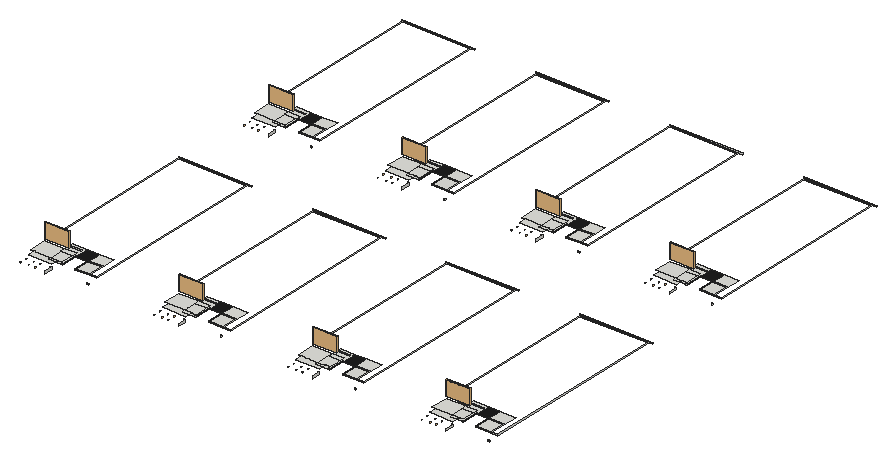
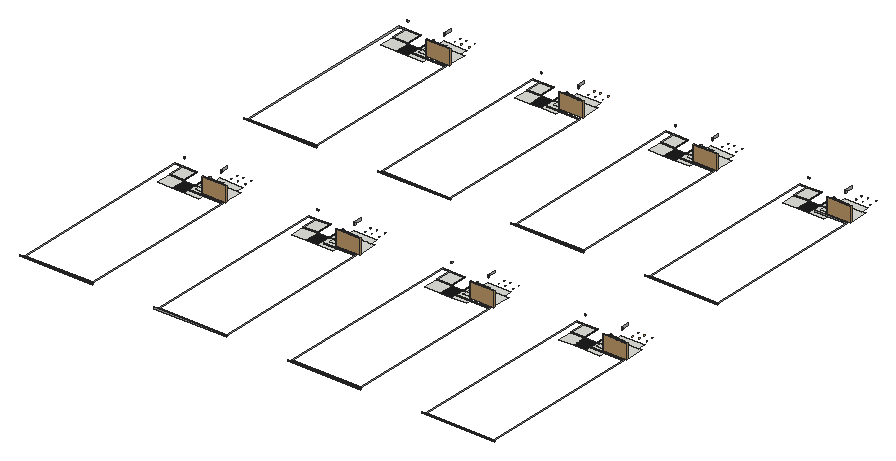
# SketchUp Ruby script. Lengths in inches.
U = 1.inch
M = Sketchup.active_model
def pt(a) = Geom::Point3d.new(a.map { |v| v * U })
def face(e, loops, mat)
  f = e.add_face(loops[0].map { |a| pt(a) })
  loops[1..].each { |l| e.add_face(l.map { |a| pt(a) }).erase! }
  f.material = f.back_material = mat if mat
  f
end
# faces: each face lists its corners as indices into pts; further lists are holes
def faces(e, pts, list, mat = nil) = list.each { |f| face(e, (f[0].is_a?(Array) ? f : [f]).map { |l| l.map { |i| pts[i] } }, mat) }
# xy, xz, yz: faces in a plane at the given z, y or x. An outline is a flat list of corners, or four numbers for a rectangle; further outlines are holes
def ring(l) = l.size == 4 ? [[l[0], l[1]], [l[2], l[1]], [l[2], l[3]], [l[0], l[3]]] : l.each_slice(2).to_a
def flat(e, list, mat, &to3) = list.each { |f| face(e, (f[0].is_a?(Array) ? f : [f]).map { |l| ring(l).map { |u, v| to3.(u, v) } }, mat) }
def xy(e, z, list, mat = nil) = flat(e, list, mat) { |x, y| [x, y, z] }
def xz(e, y, list, mat = nil) = flat(e, list, mat) { |x, z| [x, y, z] }
def yz(e, x, list, mat = nil) = flat(e, list, mat) { |y, z| [x, y, z] }
def lines(e, pts, list) = list.each { |a, b| e.add_line(pt(pts[a]), pt(pts[b])) }
# prism: a flat outline (further loops are holes) pulled along v
def prism(e, loops, v, mat = nil)
  f = face(e, loops, mat); d = Geom::Vector3d.new(v.map { |x| x * U })
  f.pushpull(f.normal.samedirection?(d) ? d.length : -d.length)
end
def box(e, o, s, mat = nil) = prism(e, [[o, [o[0] + s[0], o[1], o[2]], [o[0] + s[0], o[1] + s[1], o[2]], [o[0], o[1] + s[1], o[2]]]], [0, 0, s[2]], mat)
def at(x, y, z, deg = 0) = Geom::Transformation.translation(pt([x, y, z])) * Geom::Transformation.rotation(ORIGIN, Z_AXIS, deg.degrees)
def axes(o, x, y, z) = Geom::Transformation.new([*x, 0, *y, 0, *z, 0, *pt(o).to_a, 1])
def part(name) = M.definitions.add(name)
# library, detail: a bought-in or finely detailed component or shape, given as its bounding box
def library(name, o, s) = part(name).tap { |d| box(d.entities, o, s) }
def detail(e, o, s) = box(e.add_group.entities, o, s)
def put(e, d, t, mat = nil) = e.add_instance(d, t).tap { |i| i.material = mat if mat }
def group(e, t, mat = nil) = e.add_group.tap { |g| g.transformation = t; g.material = mat if mat }.entities
root = M.entities
M.materials.add("[Color M08]").color = [30, 30, 30]
M.materials.add("[Field Square Tile]").color = [211, 167, 108]
c1 = library("Curtains",[0,0,0],[121.73,8.19,117.22])
xy(root,252.4375,[[357.2,526.75,356.76,526.8125,356.35,526.98,356,527.25,355.74,527.6,355.57,528,355.51,528.44,355.57,528.88,355.74,529.28,356,529.63,356.35,529.9,356.76,530.07,357.2,530.13,357.63,530.07,358.04,529.9,358.39,529.63,358.66,529.28,358.83,528.88,358.88,528.44,358.83,528,358.66,527.6,358.39,527.25,358.04,526.98,357.63,526.8125],[1235.95,526.75,1235.51,526.8125,1235.1,526.98,1234.75,527.25,1234.49,527.6,1234.32,528,1234.26,528.44,1234.32,528.88,1234.49,529.28,1234.75,529.63,1235.1,529.9,1235.51,530.07,1235.95,530.13,1236.38,530.07,1236.79,529.9,1237.14,529.63,1237.41,529.28,1237.58,528.88,1237.63,528.44,1237.58,528,1237.41,527.6,1237.14,527.25,1236.79,526.98,1236.38,526.8125],[2114.7,526.75,2114.26,526.8125,2113.85,526.98,2113.5,527.25,2113.24,527.6,2113.07,528,2113.01,528.44,2113.07,528.88,2113.24,529.28,2113.5,529.63,2113.85,529.9,2114.26,530.07,2114.7,530.13,2115.13,530.07,2115.54,529.9,2115.89,529.63,2116.16,529.28,2116.33,528.88,2116.38,528.44,2116.33,528,2116.16,527.6,2115.89,527.25,2115.54,526.98,2115.13,526.8125],[2993.45,526.75,2993.01,526.8125,2992.6,526.98,2992.25,527.25,2991.99,527.6,2991.82,528,2991.76,528.44,2991.82,528.88,2991.99,529.28,2992.25,529.63,2992.6,529.9,2993.01,530.07,2993.45,530.13,2993.88,530.07,2994.29,529.9,2994.64,529.63,2994.91,529.28,2995.08,528.88,2995.13,528.44,2995.08,528,2994.91,527.6,2994.64,527.25,2994.29,526.98,2993.88,526.8125],[357.2,2362.38,356.76,2362.4375,356.35,2362.6,356,2362.87,355.74,2363.22,355.57,2363.63,355.51,2364.07,355.57,2364.5,355.74,2364.91,356,2365.26,356.35,2365.53,356.76,2365.7,357.2,2365.75,357.63,2365.7,358.04,2365.53,358.39,2365.26,358.66,2364.91,358.83,2364.5,358.88,2364.07,358.83,2363.63,358.66,2363.22,358.39,2362.87,358.04,2362.6,357.63,2362.4375],
  [1235.95,2362.38,1235.51,2362.4375,1235.1,2362.6,1234.75,2362.87,1234.49,2363.22,1234.32,2363.63,1234.26,2364.07,1234.32,2364.5,1234.49,2364.91,1234.75,2365.26,1235.1,2365.53,1235.51,2365.7,1235.95,2365.75,1236.38,2365.7,1236.79,2365.53,1237.14,2365.26,1237.41,2364.91,1237.58,2364.5,1237.63,2364.07,1237.58,2363.63,1237.41,2363.22,1237.14,2362.87,1236.79,2362.6,1236.38,2362.4375],[2114.7,2362.38,2114.26,2362.4375,2113.85,2362.6,2113.5,2362.87,2113.24,2363.22,2113.07,2363.63,2113.01,2364.07,2113.07,2364.5,2113.24,2364.91,2113.5,2365.26,2113.85,2365.53,2114.26,2365.7,2114.7,2365.75,2115.13,2365.7,2115.54,2365.53,2115.89,2365.26,2116.16,2364.91,2116.33,2364.5,2116.38,2364.07,2116.33,2363.63,2116.16,2363.22,2115.89,2362.87,2115.54,2362.6,2115.13,2362.4375],[2993.45,2362.38,2993.01,2362.4375,2992.6,2362.6,2992.25,2362.87,2991.99,2363.22,2991.82,2363.63,2991.76,2364.07,2991.82,2364.5,2991.99,2364.91,2992.25,2365.26,2992.6,2365.53,2993.01,2365.7,2993.45,2365.75,2993.88,2365.7,2994.29,2365.53,2994.64,2365.26,2994.91,2364.91,2995.08,2364.5,2995.13,2364.07,2995.08,2363.63,2994.91,2363.22,2994.64,2362.87,2994.29,2362.6,2993.88,2362.4375]],"[Field Square Tile]")
xy(root,252.5,[[266.8,476.64,266.3125,476.71,265.86,476.89,265.47,477.19,265.17,477.58,264.99,478.03,264.92,478.52,264.99,479,265.17,479.45,265.47,479.84,265.86,480.14,266.3125,480.33,266.8,480.39,267.28,480.33,267.74,480.14,268.125,479.84,268.42,479.45,268.61,479,268.67,478.52,268.61,478.03,268.42,477.58,268.125,477.19,267.74,476.89,267.28,476.71],[1145.55,476.64,1145.0625,476.71,1144.61,476.89,1144.22,477.19,1143.92,477.58,1143.74,478.03,1143.67,478.52,1143.74,479,1143.92,479.45,1144.22,479.84,1144.61,480.14,1145.0625,480.33,1145.55,480.39,1146.03,480.33,1146.49,480.14,1146.875,479.84,1147.17,479.45,1147.36,479,1147.42,478.52,1147.36,478.03,1147.17,477.58,1146.875,477.19,1146.49,476.89,1146.03,476.71],[2024.3,476.64,2023.8125,476.71,2023.36,476.89,2022.97,477.19,2022.67,477.58,2022.49,478.03,2022.42,478.52,2022.49,479,2022.67,479.45,2022.97,479.84,2023.36,480.14,2023.8125,480.33,2024.3,480.39,2024.78,480.33,2025.24,480.14,2025.625,479.84,2025.92,479.45,2026.11,479,2026.17,478.52,2026.11,478.03,2025.92,477.58,2025.625,477.19,2025.24,476.89,2024.78,476.71],[2903.05,476.64,2902.5625,476.71,2902.11,476.89,2901.72,477.19,2901.42,477.58,2901.24,478.03,2901.17,478.52,2901.24,479,2901.42,479.45,2901.72,479.84,2902.11,480.14,2902.5625,480.33,2903.05,480.39,2903.53,480.33,2903.99,480.14,2904.375,479.84,2904.67,479.45,2904.86,479,2904.92,478.52,2904.86,478.03,2904.67,477.58,2904.375,477.19,2903.99,476.89,2903.53,476.71],[317.24,479.77,316.75,479.83,316.3,480.02,315.91,480.32,315.61,480.7,315.42,481.16,315.36,481.64,315.42,482.13,315.61,482.58,315.91,482.97,316.3,483.27,316.75,483.45,317.24,483.52,317.72,483.45,318.17,483.27,318.5625,482.97,318.86,482.58,319.05,482.13,319.11,481.64,319.05,481.16,318.86,480.7,318.5625,480.32,318.17,480.02,317.72,479.83],
  [1195.99,479.77,1195.5,479.83,1195.05,480.02,1194.66,480.32,1194.36,480.7,1194.17,481.16,1194.11,481.64,1194.17,482.13,1194.36,482.58,1194.66,482.97,1195.05,483.27,1195.5,483.45,1195.99,483.52,1196.47,483.45,1196.92,483.27,1197.3125,482.97,1197.61,482.58,1197.8,482.13,1197.86,481.64,1197.8,481.16,1197.61,480.7,1197.3125,480.32,1196.92,480.02,1196.47,479.83],[2074.74,479.77,2074.25,479.83,2073.8,480.02,2073.41,480.32,2073.11,480.7,2072.92,481.16,2072.86,481.64,2072.92,482.13,2073.11,482.58,2073.41,482.97,2073.8,483.27,2074.25,483.45,2074.74,483.52,2075.22,483.45,2075.67,483.27,2076.0625,482.97,2076.36,482.58,2076.55,482.13,2076.61,481.64,2076.55,481.16,2076.36,480.7,2076.0625,480.32,2075.67,480.02,2075.22,479.83],[2953.49,479.77,2953,479.83,2952.55,480.02,2952.16,480.32,2951.86,480.7,2951.67,481.16,2951.61,481.64,2951.67,482.13,2951.86,482.58,2952.16,482.97,2952.55,483.27,2953,483.45,2953.49,483.52,2953.97,483.45,2954.42,483.27,2954.8125,482.97,2955.11,482.58,2955.3,482.13,2955.36,481.64,2955.3,481.16,2955.11,480.7,2954.8125,480.32,2954.42,480.02,2953.97,479.83],[266.8,522.58,266.3125,522.64,265.86,522.83,265.47,523.13,265.17,523.52,264.99,523.97,264.92,524.45,264.99,524.94,265.17,525.39,265.47,525.78,265.86,526.08,266.3125,526.27,266.8,526.33,267.28,526.27,267.74,526.08,268.125,525.78,268.42,525.39,268.61,524.94,268.67,524.45,268.61,523.97,268.42,523.52,268.125,523.13,267.74,522.83,267.28,522.64],[317.24,522.58,316.75,522.64,316.3,522.83,315.91,523.13,315.61,523.52,315.42,523.97,315.36,524.45,315.42,524.94,315.61,525.39,315.91,525.78,316.3,526.08,316.75,526.27,317.24,526.33,317.72,526.27,318.17,526.08,318.5625,525.78,318.86,525.39,319.05,524.94,319.11,524.45,319.05,523.97,318.86,523.52,318.5625,523.13,318.17,522.83,317.72,522.64],
  [1145.55,522.58,1145.0625,522.64,1144.61,522.83,1144.22,523.13,1143.92,523.52,1143.74,523.97,1143.67,524.45,1143.74,524.94,1143.92,525.39,1144.22,525.78,1144.61,526.08,1145.0625,526.27,1145.55,526.33,1146.03,526.27,1146.49,526.08,1146.875,525.78,1147.17,525.39,1147.36,524.94,1147.42,524.45,1147.36,523.97,1147.17,523.52,1146.875,523.13,1146.49,522.83,1146.03,522.64],[1195.99,522.58,1195.5,522.64,1195.05,522.83,1194.66,523.13,1194.36,523.52,1194.17,523.97,1194.11,524.45,1194.17,524.94,1194.36,525.39,1194.66,525.78,1195.05,526.08,1195.5,526.27,1195.99,526.33,1196.47,526.27,1196.92,526.08,1197.3125,525.78,1197.61,525.39,1197.8,524.94,1197.86,524.45,1197.8,523.97,1197.61,523.52,1197.3125,523.13,1196.92,522.83,1196.47,522.64],[2024.3,522.58,2023.8125,522.64,2023.36,522.83,2022.97,523.13,2022.67,523.52,2022.49,523.97,2022.42,524.45,2022.49,524.94,2022.67,525.39,2022.97,525.78,2023.36,526.08,2023.8125,526.27,2024.3,526.33,2024.78,526.27,2025.24,526.08,2025.625,525.78,2025.92,525.39,2026.11,524.94,2026.17,524.45,2026.11,523.97,2025.92,523.52,2025.625,523.13,2025.24,522.83,2024.78,522.64],[2074.74,522.58,2074.25,522.64,2073.8,522.83,2073.41,523.13,2073.11,523.52,2072.92,523.97,2072.86,524.45,2072.92,524.94,2073.11,525.39,2073.41,525.78,2073.8,526.08,2074.25,526.27,2074.74,526.33,2075.22,526.27,2075.67,526.08,2076.0625,525.78,2076.36,525.39,2076.55,524.94,2076.61,524.45,2076.55,523.97,2076.36,523.52,2076.0625,523.13,2075.67,522.83,2075.22,522.64],[2903.05,522.58,2902.5625,522.64,2902.11,522.83,2901.72,523.13,2901.42,523.52,2901.24,523.97,2901.17,524.45,2901.24,524.94,2901.42,525.39,2901.72,525.78,2902.11,526.08,2902.5625,526.27,2903.05,526.33,2903.53,526.27,2903.99,526.08,2904.375,525.78,2904.67,525.39,2904.86,524.94,2904.92,524.45,2904.86,523.97,2904.67,523.52,2904.375,523.13,2903.99,522.83,2903.53,522.64],
  [2953.49,522.58,2953,522.64,2952.55,522.83,2952.16,523.13,2951.86,523.52,2951.67,523.97,2951.61,524.45,2951.67,524.94,2951.86,525.39,2952.16,525.78,2952.55,526.08,2953,526.27,2953.49,526.33,2953.97,526.27,2954.42,526.08,2954.8125,525.78,2955.11,525.39,2955.3,524.94,2955.36,524.45,2955.3,523.97,2955.11,523.52,2954.8125,523.13,2954.42,522.83,2953.97,522.64],[266.8,2312.27,266.3125,2312.33,265.86,2312.52,265.47,2312.82,265.17,2313.2,264.99,2313.66,264.92,2314.14,264.99,2314.63,265.17,2315.08,265.47,2315.47,265.86,2315.77,266.3125,2315.95,266.8,2316.02,267.28,2315.95,267.74,2315.77,268.125,2315.47,268.42,2315.08,268.61,2314.63,268.67,2314.14,268.61,2313.66,268.42,2313.2,268.125,2312.82,267.74,2312.52,267.28,2312.33],[1145.55,2312.27,1145.0625,2312.33,1144.61,2312.52,1144.22,2312.82,1143.92,2313.2,1143.74,2313.66,1143.67,2314.14,1143.74,2314.63,1143.92,2315.08,1144.22,2315.47,1144.61,2315.77,1145.0625,2315.95,1145.55,2316.02,1146.03,2315.95,1146.49,2315.77,1146.875,2315.47,1147.17,2315.08,1147.36,2314.63,1147.42,2314.14,1147.36,2313.66,1147.17,2313.2,1146.875,2312.82,1146.49,2312.52,1146.03,2312.33],[2024.3,2312.27,2023.8125,2312.33,2023.36,2312.52,2022.97,2312.82,2022.67,2313.2,2022.49,2313.66,2022.42,2314.14,2022.49,2314.63,2022.67,2315.08,2022.97,2315.47,2023.36,2315.77,2023.8125,2315.95,2024.3,2316.02,2024.78,2315.95,2025.24,2315.77,2025.625,2315.47,2025.92,2315.08,2026.11,2314.63,2026.17,2314.14,2026.11,2313.66,2025.92,2313.2,2025.625,2312.82,2025.24,2312.52,2024.78,2312.33],[2903.05,2312.27,2902.5625,2312.33,2902.11,2312.52,2901.72,2312.82,2901.42,2313.2,2901.24,2313.66,2901.17,2314.14,2901.24,2314.63,2901.42,2315.08,2901.72,2315.47,2902.11,2315.77,2902.5625,2315.95,2903.05,2316.02,2903.53,2315.95,2903.99,2315.77,2904.375,2315.47,2904.67,2315.08,2904.86,2314.63,2904.92,2314.14,2904.86,2313.66,2904.67,2313.2,2904.375,2312.82,2903.99,2312.52,2903.53,2312.33],
  [317.24,2315.39,316.75,2315.46,316.3,2315.64,315.91,2315.94,315.61,2316.33,315.42,2316.78,315.36,2317.27,315.42,2317.75,315.61,2318.2,315.91,2318.59,316.3,2318.89,316.75,2319.08,317.24,2319.14,317.72,2319.08,318.17,2318.89,318.5625,2318.59,318.86,2318.2,319.05,2317.75,319.11,2317.27,319.05,2316.78,318.86,2316.33,318.5625,2315.94,318.17,2315.64,317.72,2315.46],[1195.99,2315.39,1195.5,2315.46,1195.05,2315.64,1194.66,2315.94,1194.36,2316.33,1194.17,2316.78,1194.11,2317.27,1194.17,2317.75,1194.36,2318.2,1194.66,2318.59,1195.05,2318.89,1195.5,2319.08,1195.99,2319.14,1196.47,2319.08,1196.92,2318.89,1197.3125,2318.59,1197.61,2318.2,1197.8,2317.75,1197.86,2317.27,1197.8,2316.78,1197.61,2316.33,1197.3125,2315.94,1196.92,2315.64,1196.47,2315.46],[2074.74,2315.39,2074.25,2315.46,2073.8,2315.64,2073.41,2315.94,2073.11,2316.33,2072.92,2316.78,2072.86,2317.27,2072.92,2317.75,2073.11,2318.2,2073.41,2318.59,2073.8,2318.89,2074.25,2319.08,2074.74,2319.14,2075.22,2319.08,2075.67,2318.89,2076.0625,2318.59,2076.36,2318.2,2076.55,2317.75,2076.61,2317.27,2076.55,2316.78,2076.36,2316.33,2076.0625,2315.94,2075.67,2315.64,2075.22,2315.46],[2953.49,2315.39,2953,2315.46,2952.55,2315.64,2952.16,2315.94,2951.86,2316.33,2951.67,2316.78,2951.61,2317.27,2951.67,2317.75,2951.86,2318.2,2952.16,2318.59,2952.55,2318.89,2953,2319.08,2953.49,2319.14,2953.97,2319.08,2954.42,2318.89,2954.8125,2318.59,2955.11,2318.2,2955.3,2317.75,2955.36,2317.27,2955.3,2316.78,2955.11,2316.33,2954.8125,2315.94,2954.42,2315.64,2953.97,2315.46],[266.8,2358.2,266.3125,2358.27,265.86,2358.46,265.47,2358.75,265.17,2359.14,264.99,2359.59,264.92,2360.08,264.99,2360.56,265.17,2361.02,265.47,2361.41,265.86,2361.7,266.3125,2361.89,266.8,2361.95,267.28,2361.89,267.74,2361.7,268.125,2361.41,268.42,2361.02,268.61,2360.56,268.67,2360.08,268.61,2359.59,268.42,2359.14,268.125,2358.75,267.74,2358.46,267.28,2358.27],
  [317.24,2358.2,316.75,2358.27,316.3,2358.46,315.91,2358.75,315.61,2359.14,315.42,2359.59,315.36,2360.08,315.42,2360.56,315.61,2361.02,315.91,2361.41,316.3,2361.7,316.75,2361.89,317.24,2361.95,317.72,2361.89,318.17,2361.7,318.5625,2361.41,318.86,2361.02,319.05,2360.56,319.11,2360.08,319.05,2359.59,318.86,2359.14,318.5625,2358.75,318.17,2358.46,317.72,2358.27],[1145.55,2358.2,1145.0625,2358.27,1144.61,2358.46,1144.22,2358.75,1143.92,2359.14,1143.74,2359.59,1143.67,2360.08,1143.74,2360.56,1143.92,2361.02,1144.22,2361.41,1144.61,2361.7,1145.0625,2361.89,1145.55,2361.95,1146.03,2361.89,1146.49,2361.7,1146.875,2361.41,1147.17,2361.02,1147.36,2360.56,1147.42,2360.08,1147.36,2359.59,1147.17,2359.14,1146.875,2358.75,1146.49,2358.46,1146.03,2358.27],[1195.99,2358.2,1195.5,2358.27,1195.05,2358.46,1194.66,2358.75,1194.36,2359.14,1194.17,2359.59,1194.11,2360.08,1194.17,2360.56,1194.36,2361.02,1194.66,2361.41,1195.05,2361.7,1195.5,2361.89,1195.99,2361.95,1196.47,2361.89,1196.92,2361.7,1197.3125,2361.41,1197.61,2361.02,1197.8,2360.56,1197.86,2360.08,1197.8,2359.59,1197.61,2359.14,1197.3125,2358.75,1196.92,2358.46,1196.47,2358.27],[2024.3,2358.2,2023.8125,2358.27,2023.36,2358.46,2022.97,2358.75,2022.67,2359.14,2022.49,2359.59,2022.42,2360.08,2022.49,2360.56,2022.67,2361.02,2022.97,2361.41,2023.36,2361.7,2023.8125,2361.89,2024.3,2361.95,2024.78,2361.89,2025.24,2361.7,2025.625,2361.41,2025.92,2361.02,2026.11,2360.56,2026.17,2360.08,2026.11,2359.59,2025.92,2359.14,2025.625,2358.75,2025.24,2358.46,2024.78,2358.27],[2074.74,2358.2,2074.25,2358.27,2073.8,2358.46,2073.41,2358.75,2073.11,2359.14,2072.92,2359.59,2072.86,2360.08,2072.92,2360.56,2073.11,2361.02,2073.41,2361.41,2073.8,2361.7,2074.25,2361.89,2074.74,2361.95,2075.22,2361.89,2075.67,2361.7,2076.0625,2361.41,2076.36,2361.02,2076.55,2360.56,2076.61,2360.08,2076.55,2359.59,2076.36,2359.14,2076.0625,2358.75,2075.67,2358.46,2075.22,2358.27],
  [2903.05,2358.2,2902.5625,2358.27,2902.11,2358.46,2901.72,2358.75,2901.42,2359.14,2901.24,2359.59,2901.17,2360.08,2901.24,2360.56,2901.42,2361.02,2901.72,2361.41,2902.11,2361.7,2902.5625,2361.89,2903.05,2361.95,2903.53,2361.89,2903.99,2361.7,2904.375,2361.41,2904.67,2361.02,2904.86,2360.56,2904.92,2360.08,2904.86,2359.59,2904.67,2359.14,2904.375,2358.75,2903.99,2358.46,2903.53,2358.27],[2953.49,2358.2,2953,2358.27,2952.55,2358.46,2952.16,2358.75,2951.86,2359.14,2951.67,2359.59,2951.61,2360.08,2951.67,2360.56,2951.86,2361.02,2952.16,2361.41,2952.55,2361.7,2953,2361.89,2953.49,2361.95,2953.97,2361.89,2954.42,2361.7,2954.8125,2361.41,2955.11,2361.02,2955.3,2360.56,2955.36,2360.08,2955.3,2359.59,2955.11,2359.14,2954.8125,2358.75,2954.42,2358.46,2953.97,2358.27]],"[Field Square Tile]")
xy(root,252.5625,[[357.2,481.02,356.57,481.11,355.98,481.35,355.47,481.74,355.09,482.24,354.84,482.83,354.76,483.46,354.84,484.09,355.09,484.68,355.47,485.18,355.98,485.57,356.57,485.8125,357.2,485.9,357.83,485.8125,358.42,485.57,358.92,485.18,359.31,484.68,359.55,484.09,359.63,483.46,359.55,482.83,359.31,482.24,358.92,481.74,358.42,481.35,357.83,481.11],[1235.95,481.02,1235.32,481.11,1234.73,481.35,1234.22,481.74,1233.84,482.24,1233.59,482.83,1233.51,483.46,1233.59,484.09,1233.84,484.68,1234.22,485.18,1234.73,485.57,1235.32,485.8125,1235.95,485.9,1236.58,485.8125,1237.17,485.57,1237.67,485.18,1238.06,484.68,1238.3,484.09,1238.38,483.46,1238.3,482.83,1238.06,482.24,1237.67,481.74,1237.17,481.35,1236.58,481.11],[2114.7,481.02,2114.07,481.11,2113.48,481.35,2112.97,481.74,2112.59,482.24,2112.34,482.83,2112.26,483.46,2112.34,484.09,2112.59,484.68,2112.97,485.18,2113.48,485.57,2114.07,485.8125,2114.7,485.9,2115.33,485.8125,2115.92,485.57,2116.42,485.18,2116.81,484.68,2117.05,484.09,2117.13,483.46,2117.05,482.83,2116.81,482.24,2116.42,481.74,2115.92,481.35,2115.33,481.11],[2993.45,481.02,2992.82,481.11,2992.23,481.35,2991.72,481.74,2991.34,482.24,2991.09,482.83,2991.01,483.46,2991.09,484.09,2991.34,484.68,2991.72,485.18,2992.23,485.57,2992.82,485.8125,2993.45,485.9,2994.08,485.8125,2994.67,485.57,2995.17,485.18,2995.56,484.68,2995.8,484.09,2995.88,483.46,2995.8,482.83,2995.56,482.24,2995.17,481.74,2994.67,481.35,2994.08,481.11],[357.2,2316.65,356.57,2316.73,355.98,2316.97,355.47,2317.36,355.09,2317.87,354.84,2318.45,354.76,2319.08,354.84,2319.72,355.09,2320.3,355.47,2320.81,355.98,2321.2,356.57,2321.4375,357.2,2321.52,357.83,2321.4375,358.42,2321.2,358.92,2320.81,359.31,2320.3,359.55,2319.72,359.63,2319.08,359.55,2318.45,359.31,2317.87,358.92,2317.36,358.42,2316.97,357.83,2316.73],
  [1235.95,2316.65,1235.32,2316.73,1234.73,2316.97,1234.22,2317.36,1233.84,2317.87,1233.59,2318.45,1233.51,2319.08,1233.59,2319.72,1233.84,2320.3,1234.22,2320.81,1234.73,2321.2,1235.32,2321.4375,1235.95,2321.52,1236.58,2321.4375,1237.17,2321.2,1237.67,2320.81,1238.06,2320.3,1238.3,2319.72,1238.38,2319.08,1238.3,2318.45,1238.06,2317.87,1237.67,2317.36,1237.17,2316.97,1236.58,2316.73],[2114.7,2316.65,2114.07,2316.73,2113.48,2316.97,2112.97,2317.36,2112.59,2317.87,2112.34,2318.45,2112.26,2319.08,2112.34,2319.72,2112.59,2320.3,2112.97,2320.81,2113.48,2321.2,2114.07,2321.4375,2114.7,2321.52,2115.33,2321.4375,2115.92,2321.2,2116.42,2320.81,2116.81,2320.3,2117.05,2319.72,2117.13,2319.08,2117.05,2318.45,2116.81,2317.87,2116.42,2317.36,2115.92,2316.97,2115.33,2316.73],[2993.45,2316.65,2992.82,2316.73,2992.23,2316.97,2991.72,2317.36,2991.34,2317.87,2991.09,2318.45,2991.01,2319.08,2991.09,2319.72,2991.34,2320.3,2991.72,2320.81,2992.23,2321.2,2992.82,2321.4375,2993.45,2321.52,2994.08,2321.4375,2994.67,2321.2,2995.17,2320.81,2995.56,2320.3,2995.8,2319.72,2995.88,2319.08,2995.8,2318.45,2995.56,2317.87,2995.17,2317.36,2994.67,2316.97,2994.08,2316.73]],"[Field Square Tile]")
xy(root,254.5,[[252.78,561.05,252.84,568.68],[252.84,561.05,252.84,568.68,252.78,568.68,252.78,611.02,358.39,611.02,358.39,589.83,406.85,589.83,406.85,561.05],[1131.53,561.05,1131.59,568.68],[1131.59,561.05,1131.59,568.68,1131.53,568.68,1131.53,611.02,1237.14,611.02,1237.14,589.83,1285.6,589.83,1285.6,561.05],[2010.28,561.05,2010.34,568.68],
  [2010.34,561.05,2010.34,568.68,2010.28,568.68,2010.28,611.02,2115.89,611.02,2115.89,589.83,2164.35,589.83,2164.35,561.05],[2889.03,561.05,2889.09,568.68],[2889.09,561.05,2889.09,568.68,2889.03,568.68,2889.03,611.02,2994.64,611.02,2994.64,589.83,3043.1,589.83,3043.1,561.05],[358.39,589.83,406.85,611.02],[406.85,589.83,453.7,589.83,453.7,697.21,433.97,697.21,433.97,611.02,406.85,611.02],
  [534.46,589.83,629.77,697.21],[1237.14,589.83,1285.6,611.02],[1285.6,589.83,1332.45,589.83,1332.45,697.21,1312.72,697.21,1312.72,611.02,1285.6,611.02],[1413.21,589.83,1508.52,697.21],[2115.89,589.83,2164.35,611.02],
  [2164.35,589.83,2211.2,589.83,2211.2,697.21,2191.47,697.21,2191.47,611.02,2164.35,611.02],[2291.96,589.83,2387.27,697.21],[2994.64,589.83,3043.1,611.02],[3043.1,589.83,3089.95,589.83,3089.95,697.21,3070.22,697.21,3070.22,611.02,3043.1,611.02],[3170.71,589.83,3266.02,697.21],
  [228.78,611.02,358.39,727.2],[358.39,611.02,433.97,697.21],[1107.53,611.02,1237.14,727.2],[1237.14,611.02,1312.72,697.21],[1986.28,611.02,2115.89,727.2],
  [2115.89,611.02,2191.47,697.21],[2865.03,611.02,2994.64,727.2],[2994.64,611.02,3070.22,697.21],[358.39,697.21,433.97,727.2],[433.97,697.21,453.7,697.21,453.7,792.52,358.39,792.52,358.39,727.2,433.97,727.2],
  [534.46,697.21,629.77,792.52],[1237.14,697.21,1312.72,727.2],[1312.72,697.21,1332.45,697.21,1332.45,792.52,1237.14,792.52,1237.14,727.2,1312.72,727.2],[1413.21,697.21,1508.52,792.52],[2115.89,697.21,2191.47,727.2],
  [2191.47,697.21,2211.2,697.21,2211.2,792.52,2115.89,792.52,2115.89,727.2,2191.47,727.2],[2291.96,697.21,2387.27,792.52],[2994.64,697.21,3070.22,727.2],[3070.22,697.21,3089.95,697.21,3089.95,792.52,2994.64,792.52,2994.64,727.2,3070.22,727.2],[3170.71,697.21,3266.02,792.52],
  [252.78,2396.68,252.84,2404.3],[252.84,2396.68,252.84,2404.3,252.78,2404.3,252.78,2446.65,358.39,2446.65,358.39,2425.46,406.85,2425.46,406.85,2396.68],[1131.53,2396.68,1131.59,2404.3],[1131.59,2396.68,1131.59,2404.3,1131.53,2404.3,1131.53,2446.65,1237.14,2446.65,1237.14,2425.46,1285.6,2425.46,1285.6,2396.68],[2010.28,2396.68,2010.34,2404.3],
  [2010.34,2396.68,2010.34,2404.3,2010.28,2404.3,2010.28,2446.65,2115.89,2446.65,2115.89,2425.46,2164.35,2425.46,2164.35,2396.68],[2889.03,2396.68,2889.09,2404.3],[2889.09,2396.68,2889.09,2404.3,2889.03,2404.3,2889.03,2446.65,2994.64,2446.65,2994.64,2425.46,3043.1,2425.46,3043.1,2396.68],[358.39,2425.46,406.85,2446.65],[406.85,2425.46,453.7,2425.46,453.7,2532.83,433.97,2532.83,433.97,2446.65,406.85,2446.65],
  [534.46,2425.46,629.77,2532.83],[1237.14,2425.46,1285.6,2446.65],[1285.6,2425.46,1332.45,2425.46,1332.45,2532.83,1312.72,2532.83,1312.72,2446.65,1285.6,2446.65],[1413.21,2425.46,1508.52,2532.83],[2115.89,2425.46,2164.35,2446.65],
  [2164.35,2425.46,2211.2,2425.46,2211.2,2532.83,2191.47,2532.83,2191.47,2446.65,2164.35,2446.65],[2291.96,2425.46,2387.27,2532.83],[2994.64,2425.46,3043.1,2446.65],[3043.1,2425.46,3089.95,2425.46,3089.95,2532.83,3070.22,2532.83,3070.22,2446.65,3043.1,2446.65],[3170.71,2425.46,3266.02,2532.83],
  [228.78,2446.65,358.39,2562.82],[358.39,2446.65,433.97,2532.83],[1107.53,2446.65,1237.14,2562.82],[1237.14,2446.65,1312.72,2532.83],[1986.28,2446.65,2115.89,2562.82],
  [2115.89,2446.65,2191.47,2532.83],[2865.03,2446.65,2994.64,2562.82],[2994.64,2446.65,3070.22,2532.83],[358.39,2532.83,433.97,2562.82],[433.97,2532.83,453.7,2532.83,453.7,2628.15,358.39,2628.15,358.39,2562.82,433.97,2562.82],
  [534.46,2532.83,629.77,2628.15],[1237.14,2532.83,1312.72,2562.82],[1312.72,2532.83,1332.45,2532.83,1332.45,2628.15,1237.14,2628.15,1237.14,2562.82,1312.72,2562.82],[1413.21,2532.83,1508.52,2628.15],[2115.89,2532.83,2191.47,2562.82],
  [2191.47,2532.83,2211.2,2532.83,2211.2,2628.15,2115.89,2628.15,2115.89,2562.82,2191.47,2562.82],[2291.96,2532.83,2387.27,2628.15],[2994.64,2532.83,3070.22,2562.82],[3070.22,2532.83,3089.95,2532.83,3089.95,2628.15,2994.64,2628.15,2994.64,2562.82,3070.22,2562.82],[3170.71,2532.83,3266.02,2628.15]])
xy(root,254.5,[[453.7,697.21,534.46,792.52],[1332.45,697.21,1413.21,792.52],[2211.2,697.21,2291.96,792.52],[3089.95,697.21,3170.71,792.52],[453.7,2532.83,534.46,2628.15],
  [1332.45,2532.83,1413.21,2628.15],[2211.2,2532.83,2291.96,2628.15],[3089.95,2532.83,3170.71,2628.15]],"[Color M08]")
xz(root,511.08,[[433.97,254.5,442.35,270.8125],[676.54,254.5,677.98,260.5],[677.98,254.5,686.35,260.5],[1312.72,254.5,1321.1,270.8125],[1555.29,254.5,1556.73,260.5],
  [1556.73,254.5,1565.1,260.5],[2191.47,254.5,2199.85,270.8125],[2434.04,254.5,2435.48,260.5],[2435.48,254.5,2443.85,260.5],[3070.22,254.5,3078.6,270.8125],
  [3312.79,254.5,3314.23,260.5],[3314.23,254.5,3322.6,260.5]])
xz(root,589.83,[[444.78,254.5,453.7,260.5],[534.46,254.5,629.77,260.5],[629.77,254.5,676.54,260.5],[1323.53,254.5,1332.45,260.5],[1413.21,254.5,1508.52,260.5],
  [1508.52,254.5,1555.29,260.5],[2202.28,254.5,2211.2,260.5],[2291.96,254.5,2387.27,260.5],[2387.27,254.5,2434.04,260.5],[3081.03,254.5,3089.95,260.5],
  [3170.71,254.5,3266.02,260.5],[3266.02,254.5,3312.79,260.5]])
xz(root,697.21,[[534.46,254.5,629.77,260.5],[1413.21,254.5,1508.52,260.5],[2291.96,254.5,2387.27,260.5],[3170.71,254.5,3266.02,260.5]])
xz(root,762.17,[[228.78,254.5,444.78,260.5],[1107.53,254.5,1323.53,260.5],[1986.28,254.5,2202.28,260.5],[2865.03,254.5,3081.03,260.5]])
xz(root,1825.82,[[228.78,254.5,676.54,260.5],[1107.53,254.5,1555.29,260.5],[1986.28,254.5,2434.04,260.5],[2865.03,254.5,3312.79,260.5]])
xz(root,1835.625,[[218.97,254.5,698.16,260.5],[1097.72,254.5,1576.91,260.5],[1976.47,254.5,2455.66,260.5],[2855.22,254.5,3334.41,260.5]])
xz(root,2346.71,[[433.97,254.5,442.35,270.8125],[676.54,254.5,677.98,260.5],[677.98,254.5,686.35,260.5],[1312.72,254.5,1321.1,270.8125],[1555.29,254.5,1556.73,260.5],
  [1556.73,254.5,1565.1,260.5],[2191.47,254.5,2199.85,270.8125],[2434.04,254.5,2435.48,260.5],[2435.48,254.5,2443.85,260.5],[3070.22,254.5,3078.6,270.8125],
  [3312.79,254.5,3314.23,260.5],[3314.23,254.5,3322.6,260.5]])
xz(root,2425.46,[[444.78,254.5,453.7,260.5],[534.46,254.5,629.77,260.5],[629.77,254.5,676.54,260.5],[1323.53,254.5,1332.45,260.5],[1413.21,254.5,1508.52,260.5],
  [1508.52,254.5,1555.29,260.5],[2202.28,254.5,2211.2,260.5],[2291.96,254.5,2387.27,260.5],[2387.27,254.5,2434.04,260.5],[3081.03,254.5,3089.95,260.5],
  [3170.71,254.5,3266.02,260.5],[3266.02,254.5,3312.79,260.5]])
xz(root,2532.83,[[534.46,254.5,629.77,260.5],[1413.21,254.5,1508.52,260.5],[2291.96,254.5,2387.27,260.5],[3170.71,254.5,3266.02,260.5]])
xz(root,2597.8,[[228.78,254.5,444.78,260.5],[1107.53,254.5,1323.53,260.5],[1986.28,254.5,2202.28,260.5],[2865.03,254.5,3081.03,260.5]])
xz(root,3661.44,[[228.78,254.5,676.54,260.5],[1107.53,254.5,1555.29,260.5],[1986.28,254.5,2434.04,260.5],[2865.03,254.5,3312.79,260.5]])
xz(root,3671.25,[[218.97,254.5,698.16,260.5],[1097.72,254.5,1576.91,260.5],[1976.47,254.5,2455.66,260.5],[2855.22,254.5,3334.41,260.5]])
yz(root,228.78,[[762.17,254.5,1825.82,260.5],[2597.8,254.5,3661.44,260.5]])
yz(root,442.35,[[458.5,254.5,511.08,270.8125],[2294.125,254.5,2346.71,270.8125]])
yz(root,453.7,[[589.83,254.5,697.21,260.5],[2425.46,254.5,2532.83,260.5]],"[Color M08]")
yz(root,534.46,[[589.83,254.5,697.21,260.5],[2425.46,254.5,2532.83,260.5]],"[Color M08]")
yz(root,629.77,[[589.83,254.5,697.21,260.5],[2425.46,254.5,2532.83,260.5]])
yz(root,676.54,[[589.83,254.5,1825.82,260.5],[2425.46,254.5,3661.44,260.5]])
yz(root,1107.53,[[762.17,254.5,1825.82,260.5],[2597.8,254.5,3661.44,260.5]])
yz(root,1321.1,[[458.5,254.5,511.08,270.8125],[2294.125,254.5,2346.71,270.8125]])
yz(root,1332.45,[[589.83,254.5,697.21,260.5],[2425.46,254.5,2532.83,260.5]],"[Color M08]")
yz(root,1413.21,[[589.83,254.5,697.21,260.5],[2425.46,254.5,2532.83,260.5]],"[Color M08]")
yz(root,1508.52,[[589.83,254.5,697.21,260.5],[2425.46,254.5,2532.83,260.5]])
yz(root,1555.29,[[589.83,254.5,1825.82,260.5],[2425.46,254.5,3661.44,260.5]])
yz(root,1986.28,[[762.17,254.5,1825.82,260.5],[2597.8,254.5,3661.44,260.5]])
yz(root,2199.85,[[458.5,254.5,511.08,270.8125],[2294.125,254.5,2346.71,270.8125]])
yz(root,2211.2,[[589.83,254.5,697.21,260.5],[2425.46,254.5,2532.83,260.5]],"[Color M08]")
yz(root,2291.96,[[589.83,254.5,697.21,260.5],[2425.46,254.5,2532.83,260.5]],"[Color M08]")
yz(root,2387.27,[[589.83,254.5,697.21,260.5],[2425.46,254.5,2532.83,260.5]])
yz(root,2434.04,[[589.83,254.5,1825.82,260.5],[2425.46,254.5,3661.44,260.5]])
yz(root,2865.03,[[762.17,254.5,1825.82,260.5],[2597.8,254.5,3661.44,260.5]])
yz(root,3078.6,[[458.5,254.5,511.08,270.8125],[2294.125,254.5,2346.71,270.8125]])
yz(root,3089.95,[[589.83,254.5,697.21,260.5],[2425.46,254.5,2532.83,260.5]],"[Color M08]")
yz(root,3170.71,[[589.83,254.5,697.21,260.5],[2425.46,254.5,2532.83,260.5]],"[Color M08]")
yz(root,3266.02,[[589.83,254.5,697.21,260.5],[2425.46,254.5,2532.83,260.5]])
yz(root,3312.79,[[589.83,254.5,1825.82,260.5],[2425.46,254.5,3661.44,260.5]])
put(root,c1,axes([1974.85,739.17,259.59],[1.29555,0,0],[0,1,0],[0,0,0.8242]))
put(root,c1,axes([2853.6,739.17,259.59],[1.29555,0,0],[0,1,0],[0,0,0.8242]))
put(root,c1,axes([1096.1,739.17,259.59],[1.29555,0,0],[0,1,0],[0,0,0.8242]))
put(root,c1,axes([217.35,739.17,259.59],[1.29555,0,0],[0,1,0],[0,0,0.8242]))
put(root,c1,axes([1096.1,2574.79,259.59],[1.29555,0,0],[0,1,0],[0,0,0.8242]))
put(root,c1,axes([2853.6,2574.79,259.59],[1.29555,0,0],[0,1,0],[0,0,0.8242]))
put(root,c1,axes([1974.85,2574.79,259.59],[1.29555,0,0],[0,1,0],[0,0,0.8242]))
put(root,c1,axes([217.35,2574.79,259.59],[1.29555,0,0],[0,1,0],[0,0,0.8242]))
